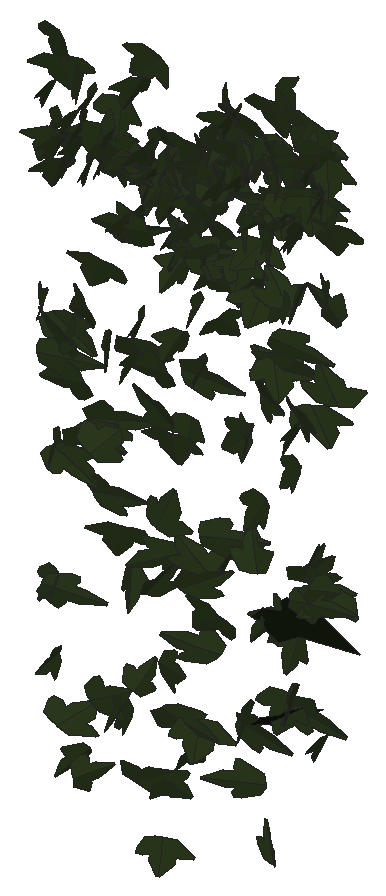
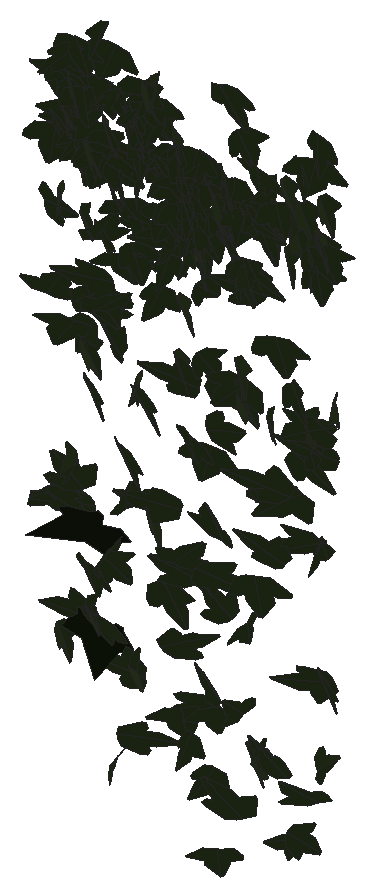
# SketchUp Ruby script. Lengths in millimetres.
U = 1.mm
M = Sketchup.active_model
def pt(a) = Geom::Point3d.new(a.map { |v| v * U })
def face(e, loops, mat)
  f = e.add_face(loops[0].map { |a| pt(a) })
  loops[1..].each { |l| e.add_face(l.map { |a| pt(a) }).erase! }
  f.material = f.back_material = mat if mat
  f
end
# faces: each face lists its corners as indices into pts; further lists are holes
def faces(e, pts, list, mat = nil) = list.each { |f| face(e, (f[0].is_a?(Array) ? f : [f]).map { |l| l.map { |i| pts[i] } }, mat) }
# xy, xz, yz: faces in a plane at the given z, y or x. An outline is a flat list of corners, or four numbers for a rectangle; further outlines are holes
def ring(l) = l.size == 4 ? [[l[0], l[1]], [l[2], l[1]], [l[2], l[3]], [l[0], l[3]]] : l.each_slice(2).to_a
def flat(e, list, mat, &to3) = list.each { |f| face(e, (f[0].is_a?(Array) ? f : [f]).map { |l| ring(l).map { |u, v| to3.(u, v) } }, mat) }
def xy(e, z, list, mat = nil) = flat(e, list, mat) { |x, y| [x, y, z] }
def xz(e, y, list, mat = nil) = flat(e, list, mat) { |x, z| [x, y, z] }
def yz(e, x, list, mat = nil) = flat(e, list, mat) { |y, z| [x, y, z] }
def lines(e, pts, list) = list.each { |a, b| e.add_line(pt(pts[a]), pt(pts[b])) }
# prism: a flat outline (further loops are holes) pulled along v
def prism(e, loops, v, mat = nil)
  f = face(e, loops, mat); d = Geom::Vector3d.new(v.map { |x| x * U })
  f.pushpull(f.normal.samedirection?(d) ? d.length : -d.length)
end
def box(e, o, s, mat = nil) = prism(e, [[o, [o[0] + s[0], o[1], o[2]], [o[0] + s[0], o[1] + s[1], o[2]], [o[0], o[1] + s[1], o[2]]]], [0, 0, s[2]], mat)
def at(x, y, z, deg = 0) = Geom::Transformation.translation(pt([x, y, z])) * Geom::Transformation.rotation(ORIGIN, Z_AXIS, deg.degrees)
def axes(o, x, y, z) = Geom::Transformation.new([*x, 0, *y, 0, *z, 0, *pt(o).to_a, 1])
def part(name) = M.definitions.add(name)
# library, detail: a bought-in or finely detailed component or shape, given as its bounding box
def library(name, o, s) = part(name).tap { |d| box(d.entities, o, s) }
def detail(e, o, s) = box(e.add_group.entities, o, s)
def put(e, d, t, mat = nil) = e.add_instance(d, t).tap { |i| i.material = mat if mat }
def group(e, t, mat = nil) = e.add_group.tap { |g| g.transformation = t; g.material = mat if mat }.entities
root = M.entities
M.materials.add("efeu1").color = [18, 25, 13]
M.materials.add("efeu2").color = [43, 57, 29]
c1 = part("ivyleaf_10")
p = [[0,12.8,-0.8],[-1.5,51.3,-10.9],[-4.9,51,-11.6],[-13.6,26.5,-7.3],[-13.2,15.9,-4.6],[-21.1,19.3,-7.2],
  [-29.5,16.3,-8.3],[-29.2,8.3,-6.2],[-19.7,-9.8,0.5],[-7.6,-13,4],[1,-12.2,5.8],[-0.4,51.1,-11.1],
  [-1.5,51.1,-10.9],[1,-12.4,5.9],[16.9,-12.4,3.5],[35.1,9.1,-5.1],[35,12.9,-6.1],[20.5,16.4,-4.9],
  [15.8,15,-3.8],[15.3,27.6,-7.1],[12.8,31.3,-7.8]]
faces(c1.entities,p,[[0,1,2,3,4,5,6,7,8,9,10],[11,12,0,13,14,15,16,17,18,19,20]],"efeu2")
c2 = part("ivyleaf_9")
p = [[39.1,54.8,31.7],[34.5,51.8,30.2],[-5.3,25.2,17.3],[-17.9,28.3,20.9],[-21.6,21.7,17],[-20.2,4.3,5.3],
  [-22.9,-0.3,2.5],[-17.1,-4,-0.6],[-2,-2.1,-1.2],[-0.7,-15.4,-10.1],[16.6,-22.3,-16.7],[21.1,-15.1,-12.5],
  [32.7,-10.7,-11],[46.1,-1.8,-6.6],[30.8,11.2,3.8]]
faces(c2.entities,p,[[0,1,2,3,4,5,6,7,8,9,10,11,12,13,14]],"efeu1")
put(root,c1,axes([1332.3,1036.5,560.2],[-0.00686,-0.08927,-0.63569],[-0.05798,0.635,-0.089],[1.22033,0.02967,-0.0078]))
put(root,c1,axes([1336.2,1057.5,753.6],[-0.73583,-0.46937,0.22543],[-0.14974,-0.22489,-0.6032],[0.97962,-0.38694,0.07713]))
put(root,c1,axes([1332.1,1056.3,814.7],[0.09283,-0.6554,-0.01014],[-0.00037,0.01015,-0.65721],[1.2475,0.04877,0.00056]))
put(root,c1,axes([1331.9,1063.9,125.8],[-0.04625,0.08812,-0.63188],[-0.26385,-0.61795,-0.08085],[-1.18521,0.13413,0.04265]))
put(root,c1,axes([1332.8,1054.4,227.3],[0.67152,-0.55596,-0.04211],[-0.04288,0.03558,-0.65847],[1.06026,0.35356,0.00004]))
put(root,c1,axes([1336.6,1057.8,771.8],[0.39508,-0.57519,-0.19],[-0.0814,0.18643,-0.61111],[1.15,0.2108,0.02202]))
put(root,c1,axes([1343.5,1052.7,726],[-0.47128,-0.6144,-0.03144],[0.02093,0.02946,-0.66242],[1.17066,-0.24787,-0.00081]))
put(root,c1,axes([1340.5,1050.9,389.7],[0.17693,-0.48285,-0.47024],[0.2146,0.47915,-0.4697],[1.26468,-0.01375,0.14549]))
put(root,c1,axes([1347.1,1047.8,757],[-0.15632,-0.66371,0.02105],[-0.00056,-0.02118,-0.66877],[1.26381,-0.08211,0.00231]))
put(root,c1,axes([1346.4,1044.7,881.1],[0.93655,-0.44172,-0.14903],[0.10035,0.26804,-0.62036],[0.88154,0.43877,0.22895]))
put(root,c1,axes([1367.5,1039.1,522.4],[-0.44439,0.33408,-0.55742],[-0.77806,0.38491,0.40194],[0.96143,0.46592,0.06763]))
put(root,c1,axes([1352.7,1048.3,851.2],[-1.13155,-0.29765,-0.08444],[0.17649,0.00307,-0.66378],[0.56176,-0.60051,0.03846]))
put(root,c1,axes([1375.6,1043.5,480.4],[-0.57648,0.07771,0.61393],[-1.16722,0.05355,-0.30936],[-0.15721,-0.68249,0.04563]))
put(root,c1,axes([1354.8,1052.8,738.9],[0.38297,-0.5402,-0.28923],[0.00625,0.30537,-0.56806],[1.16617,0.17576,0.09803]))
put(root,c1,axes([1358.2,1045.3,518.6],[0.63988,-0.5789,0.1251],[-0.11321,0.11013,0.66944],[-1.12151,-0.34141,0.00381]))
put(root,c1,axes([1365.8,1049.1,792.1],[-0.02554,-0.65638,0.0168],[-0.01007,-0.01669,-0.6565],[1.2496,-0.01355,-0.00495]))
put(root,c1,axes([1366.6,1061.7,25.4],[-0.0766,-0.43309,0.47651],[-0.0449,-0.47613,-0.43473],[1.22468,-0.04454,0.01386]))
put(root,c1,axes([1341.7,1048.7,220.6],[-0.28811,-0.09888,-0.63937],[1.1804,0.16469,-0.17232],[0.35041,-0.63607,0.05477]))
put(root,c1,axes([1343.2,1056.3,534.8],[0.90612,0.09577,0.47932],[0.86018,0.16854,-0.48261],[-0.35425,0.65422,0.05416]))
put(root,c1,axes([1339.2,1046.5,498.4],[0.19337,-0.05206,-0.67101],[1.27587,-0.0523,0.10556],[-0.11349,-0.67664,0.04347]))
put(root,c1,axes([1381,1050.2,566.6],[-0.56102,0.23975,0.51389],[-0.84038,0.26634,-0.37754],[-0.67714,-0.52919,0.0428]))
put(root,c1,axes([1372.9,1050.3,761.5],[-0.05381,-0.65385,-0.01163],[-0.01269,0.01193,-0.65443],[1.24455,-0.02815,-0.00717]))
put(root,c1,axes([1357.6,1045.7,68.6],[0.87358,0.11605,-0.44595],[0.67555,0.31233,0.44663],[0.55924,-0.55857,0.15709]))
put(root,c1,axes([1354.6,1044.4,385.3],[0.79663,0.19512,0.47103],[0.81579,0.19531,-0.46181],[-0.52541,0.59911,-0.00286]))
put(root,c1,axes([1377.4,1043.1,841.4],[0.54888,-0.57359,-0.24048],[-0.04153,0.25558,-0.63578],[1.18299,0.27511,0.08925]))
put(root,c1,axes([1380.4,1041.2,787],[-0.03679,-0.49141,-0.47177],[0.08739,0.46995,-0.49139],[1.29354,-0.04572,0.01978]))
put(root,c1,axes([1380.1,1057.1,736.3],[0.28652,-0.62247,-0.10999],[0.05396,0.1196,-0.63806],[1.20182,0.14303,0.05487]))
put(root,c1,axes([1383.4,1056.8,819],[0.25412,-0.64214,-0.01462],[-0.01335,0.01347,-0.65586],[1.22237,0.13364,-0.00412]))
put(root,c1,axes([1397.3,1056.8,620.3],[-1.15263,-0.08738,0.19608],[-0.36259,-0.05166,-0.61147],[0.18826,-0.63448,0.02279]))
put(root,c1,axes([1379,1044.6,11.4],[0.07847,0.04993,-0.655],[0.61551,0.5697,0.06379],[1.0882,-0.32583,0.01115]))
put(root,c1,axes([1398.4,1053.5,783.8],[-0.78386,-0.51185,0.09508],[0.05626,-0.14403,-0.64733],[0.98922,-0.3974,0.11216]))
put(root,c1,axes([1388.5,1040.3,427],[-0.79844,-0.26297,-0.51972],[0.84591,0.26942,-0.4951],[0.71645,-0.61117,0.00537]))
put(root,c1,axes([1406.6,1044.4,758],[0.3273,-0.5681,-0.25628],[0.01322,0.26759,-0.58851],[1.18607,0.15379,0.07728]))
put(root,c1,axes([1398.6,1065.4,528.8],[0.425,-0.52002,0.29566],[0.40747,-0.2252,-0.5578],[1.06306,0.29422,0.0956]))
put(root,c1,axes([1416.6,1053.4,753.1],[0.87223,-0.29069,-0.36046],[-0.32277,0.36655,-0.51122],[0.82009,0.45344,0.18218]))
put(root,c1,axes([1392.2,1060.8,99.8],[0.82859,-0.19174,-0.44873],[0.762,-0.20342,0.47538],[-0.53093,-0.59121,-0.01803]))
put(root,c1,axes([1407.6,1035,417.3],[0.55694,0.2796,-0.64011],[0.62537,0.55732,0.39366],[1.17312,-0.42984,0.09404]))
put(root,c1,axes([1442.8,1055.9,764.5],[-0.12836,0.12528,0.62325],[-1.2046,0.04537,-0.07761],[-0.11313,-0.62524,0.11925]))
put(root,c1,axes([1427.5,1055.3,313.8],[-1.04517,-0.37019,0.07828],[-0.12379,-0.04356,-0.66228],[0.7094,-0.553,-0.00024]))
put(root,c1,axes([1401.5,1053.4,438.2],[-0.36839,-0.16323,0.66632],[0.98798,0.41776,0.25314],[-0.85356,0.554,0.00543]))
put(root,c1,axes([1421.4,1034.9,796.7],[-0.02991,-0.03598,-0.69138],[0.26434,0.67733,-0.03841],[1.29082,-0.13954,-0.00815]))
put(root,c1,axes([1420.3,1058.6,100],[0.15907,-0.19679,0.62358],[0.39507,-0.58815,-0.21343],[1.18012,0.22342,-0.0126]))
put(root,c1,axes([1404.6,1049.6,353.1],[-0.50568,-0.03052,0.58921],[1.10998,0.08414,0.26735],[-0.16981,0.64085,-0.00704]))
put(root,c1,axes([1422,1044.4,777.7],[-0.68013,-0.43856,-0.36402],[0.43322,0.28409,-0.56572],[0.99447,-0.42369,-0.00252]))
put(root,c1,axes([1435.2,1052.3,102.8],[0.50005,-0.5423,-0.26097],[-0.20438,0.23794,-0.60257],[1.12702,0.28377,0.00652]))
put(root,c1,axes([1455.3,1045.9,687.6],[-0.41925,-0.00398,0.66367],[-1.25886,-0.05607,-0.21989],[0.10366,-0.69702,0.0139]))
put(root,c1,axes([1423.7,1052.5,821.2],[1.16308,-0.26994,0.16014],[0.26839,-0.07699,-0.66795],[0.53365,0.62704,-0.01308]))
put(root,c1,axes([1438.9,1052.8,691],[-0.23653,-0.64738,-0.0655],[0.01686,0.065,-0.65919],[1.23826,-0.12454,-0.00354]))
put(root,c1,axes([1415,1049.3,757.9],[-0.44416,0.07954,-0.60477],[1.06648,-0.22786,-0.2462],[-0.45865,-0.60687,0.01317]))
put(root,c1,axes([1437,1059.4,261.7],[0.12007,0.64123,-0.31004],[-0.1205,-0.30497,-0.64364],[-1.35019,0.08424,0.02987]))
put(root,c1,axes([1443.5,1055.1,698],[-0.32129,-0.60605,-0.25],[0.13768,0.23936,-0.6291],[1.24009,-0.18359,0.00507]))
put(root,c1,axes([1447.6,1053.3,856.4],[-0.33131,-0.62171,0.15575],[-0.02896,-0.15734,-0.64506],[1.21946,-0.17265,0.027]))
put(root,c1,axes([1443.3,1054.2,760.9],[-0.74897,-0.50942,-0.15101],[0.27774,0.07706,-0.64027],[0.97234,-0.4144,0.06657]))
put(root,c1,axes([1446.6,1052.1,531],[0.15266,-0.60947,0.22363],[0.04973,-0.22211,-0.61472],[1.23457,0.08431,-0.00289]))
put(root,c1,axes([1449.3,1055.5,574.8],[0.20397,-0.62045,-0.16683],[-0.01936,0.16748,-0.62939],[1.22263,0.10616,0.01786]))
put(root,c1,axes([1431.4,1052.7,672],[-0.11162,-0.34172,0.53698],[0.67526,0.43015,0.31248],[-1.0057,0.32674,0.15022]))
put(root,c1,axes([1452.9,1047.3,143.9],[0.30692,0.38769,-0.48276],[0.37266,0.44133,0.41983],[1.11791,-0.25356,-0.00741]))
put(root,c1,axes([1461.6,1055.5,742.7],[0.36603,-0.6045,-0.13853],[0.06646,0.15536,-0.62948],[1.17844,0.179,0.07853]))
put(root,c1,axes([1452.5,1048.8,546.1],[-1.19271,0.08538,-0.31229],[0.58647,-0.05139,-0.63242],[-0.18898,-0.6983,0.00836]))
put(root,c1,axes([1463.7,1045.1,786.7],[-0.29152,-0.57233,-0.33623],[0.17215,0.32385,-0.59247],[1.25154,-0.17786,0.00318]))
put(root,c1,axes([1469.3,1059.9,750.2],[-0.58038,-0.55748,0.12489],[0.01226,-0.14492,-0.63113],[1.08722,-0.29596,0.07379]))
put(root,c1,axes([1462.9,1063.4,734.3],[0.74107,-0.48932,0.14193],[0.16888,-0.11077,-0.62534],[0.95484,0.39936,0.00045]))
put(root,c1,axes([1488.6,1041.8,533],[-0.50398,0.0617,0.60507],[-1.13825,0.09356,-0.27128],[-0.21044,-0.65382,0.01827]))
put(root,c1,axes([1469.7,1054.8,793.7],[0.41106,-0.59554,-0.18444],[-0.0672,0.1832,-0.63287],[1.18463,0.21704,0.0281]))
put(root,c1,axes([1474.9,1044.3,897.7],[1.05169,-0.26567,-0.34608],[-0.45899,0.2794,-0.59957],[0.69197,0.58912,0.12829]))
put(root,c1,axes([1472.4,1057.6,752.4],[-0.3491,-0.62597,0.04653],[-0.03518,-0.04307,-0.65227],[1.19411,-0.18427,-0.00561]))
put(root,c1,axes([1455.2,1056,26],[-0.92702,-0.19327,0.39528],[0.70381,0.13972,0.524],[-0.45377,0.61154,0.00521]))
put(root,c1,axes([1491.8,1042.2,476.2],[-0.53705,0.20796,-0.5476],[-0.81467,0.34171,0.35035],[0.76099,0.51257,-0.01139]))
put(root,c1,axes([1476.1,1057.9,767.1],[0.10141,-0.6501,-0.05822],[-0.01499,0.05777,-0.65228],[1.24214,0.05377,-0.00312]))
put(root,c1,axes([1480.4,1055.4,749.7],[-0.79794,-0.40959,0.25796],[-0.15047,-0.27875,-0.57109],[0.90888,-0.40574,0.13193]))
put(root,c1,axes([1489.1,1059.7,306.5],[-0.42664,-0.25606,0.61545],[-0.58968,-0.53489,-0.3354],[1.12328,-0.37805,0.05768]))
put(root,c1,axes([1472.2,1051.6,262.5],[-0.14374,-0.60993,0.28193],[0.0693,0.27957,0.61458],[-1.27695,0.08383,0.00162]))
put(root,c1,axes([1487.9,1063.3,728.6],[-0.30697,-0.60038,0.14721],[-0.03151,-0.14788,-0.62129],[1.17607,-0.16067,0.02178]))
put(root,c1,axes([1482.5,1051,-39.4],[0.8563,0.44593,-0.07956],[-0.11736,-0.0508,-0.63343],[-0.85408,0.45408,0.00727]))
put(root,c1,axes([1492.7,1052.8,783.8],[0.45627,-0.59477,0.09252],[0.04733,-0.08971,-0.64118],[1.14459,0.2408,-0.01037]))
put(root,c1,axes([1477.4,1065.7,166.1],[0.16267,-0.18588,-0.63532],[0.62281,-0.54498,0.20348],[-1.09513,-0.33754,0.02135]))
put(root,c1,axes([1495.9,1051.3,450.6],[-1.21277,-0.02421,-0.01622],[0.03089,-0.00002,-0.63769],[0.04606,-0.63743,0.00063]))
put(root,c1,axes([1496.1,1054.8,740.2],[0.35355,-0.58758,-0.16925],[0.01696,0.17947,-0.61328],[1.16362,0.17591,0.06036]))
put(root,c1,axes([1486.8,1046.2,351.5],[1.20432,-0.35767,-0.06101],[0.11766,-0.01458,0.72666],[-0.68045,-0.63555,0.01767]))
put(root,c1,axes([1497.5,1057.8,568.8],[-0.27937,-0.50179,0.37147],[0.09764,-0.39,-0.50655],[1.18419,-0.08622,0.1294]))
put(root,c1,axes([1498.9,1057.2,655.8],[-0.31972,-0.36698,0.51188],[0.22237,-0.53874,-0.34789],[1.1779,0.0021,0.20462]))
put(root,c1,axes([1502.4,1047,702.2],[0.06894,-0.59354,-0.25176],[0.05631,0.25342,-0.5932],[1.22575,0.02174,0.04141]))
put(root,c1,axes([1495.5,1051.9,806.6],[-0.98716,0.3402,-0.19325],[0.29031,-0.11968,-0.6201],[-0.68572,-0.54042,0.01567]))
put(root,c1,axes([1502,1041.8,793.2],[0.36663,0.60685,0.10715],[-0.20021,0.143,-0.62076],[-1.15562,0.16775,0.14154]))
put(root,c1,axes([1499.7,1040.5,47],[-0.43307,-0.44365,-0.43111],[0.45879,0.35945,-0.49714],[1.08427,-0.32929,0.03816]))
put(root,c1,axes([1500.4,1046.2,792.3],[-0.03249,0.63833,-0.12351],[0.02033,-0.12326,-0.63852],[-1.23723,-0.01879,-0.00725]))
put(root,c1,axes([1509.9,1050.3,686.3],[0.39484,-0.57715,-0.18427],[-0.06742,0.18289,-0.61269],[1.15108,0.20868,0.02732]))
put(root,c1,axes([1510.6,1036.9,672.9],[0.51034,-0.36345,0.57601],[-0.45291,0.53003,0.44522],[-1.21455,-0.35037,0.076]))
put(root,c1,axes([1506.3,1054,776.9],[1.22294,0.11943,0.00816],[-0.00731,0.0651,-0.65037],[-0.22771,0.63932,0.0647]))
put(root,c1,axes([1509.8,1059.3,761.6],[0.81436,-0.48623,0.05749],[0.15634,-0.00397,-0.64502],[0.91863,0.43172,0.05881]))
put(root,c1,axes([1517.3,1050.3,807.3],[-1.18894,0.18782,0.04065],[-0.07439,0.0112,-0.65233],[-0.35809,-0.62593,0.00053]))
put(root,c1,axes([1507.1,1063.3,465.6],[1.02582,-0.35639,0.20084],[0.31834,-0.11118,-0.64617],[0.71051,0.56436,-0.00046]))
put(root,c1,axes([1522.2,1050.4,741],[-1.02527,0.31995,0.11542],[-0.24543,0.00792,-0.62386],[-0.59901,-0.55088,0.05806]))
put(root,c1,axes([1532.3,1064.2,205.3],[0.27797,0.31587,0.61204],[-0.55052,-0.53967,0.34754],[1.18961,-0.32355,0.01782]))
put(root,c1,axes([1503.6,1042.7,128.8],[-0.82742,-0.05458,-0.5217],[0.97999,0.08485,-0.43797],[0.19044,-0.67378,-0.0129]))
put(root,c1,axes([1520.6,1051.7,86.5],[-0.1856,-0.47273,-0.46587],[0.22044,0.45153,-0.48242],[1.24379,-0.15057,0.01598]))
put(root,c1,axes([1522.5,1058,758.1],[0.52452,-0.58774,-0.07754],[0.02356,0.0912,-0.64726],[1.12804,0.27138,0.04957]))
put(root,c1,axes([1537.9,1041.9,690.6],[0.95335,0.00863,0.51223],[-0.96947,0.08467,0.49672],[-0.10382,-0.71143,0.06533]))
put(root,c1,axes([1521.3,1057.7,777.2],[1.0362,0.33969,-0.08162],[-0.15284,-0.02539,-0.64139],[-0.64709,0.54995,0.0208]))
put(root,c1,axes([1529.9,1057.6,308.8],[0.80325,0.40958,0.25548],[-0.34746,-0.17872,0.58812],[0.85049,-0.45985,-0.00102]))
put(root,c1,axes([1524.2,1049.2,688],[0.09501,-0.38401,-0.51185],[0.1175,0.5139,-0.37953],[1.21214,-0.01972,0.07691]))
put(root,c1,axes([1524.3,1042.8,716],[-0.39327,-0.53988,-0.30294],[0.25629,0.27252,-0.57753],[1.14999,-0.24536,0.02511]))
put(root,c1,axes([1529.4,1058.6,740.2],[-0.74614,-0.51318,0.08154],[0.06449,-0.12718,-0.63748],[0.98682,-0.3797,0.10331]))
put(root,c1,axes([1528.5,1053.8,621.7],[0.42056,-0.60664,-0.00253],[-0.00166,0.00238,-0.64563],[1.15457,0.22098,-0.00001]))
put(root,c1,axes([1532.1,1053.3,793.2],[-0.27681,-0.63951,0.10688],[0.00076,-0.10962,-0.65539],[1.23399,-0.14339,0.02438]))
put(root,c1,axes([1538.9,1052.5,803.4],[-0.76857,0.39671,0.35406],[-0.5682,0.19874,-0.5632],[-0.83742,-0.49894,0.05718]))
put(root,c1,axes([1535.1,1054.3,762.3],[-1.08496,-0.29009,0.06256],[-0.09396,-0.0409,-0.63948],[0.55692,-0.57204,0.01399]))
put(root,c1,axes([1536.9,1046.4,783.6],[-1.21714,-0.08182,0.08241],[-0.13865,-0.07655,-0.64133],[0.17211,-0.64025,0.06615]))
put(root,c1,axes([1535.1,1051.9,550.5],[0.29222,-0.61507,-0.08584],[-0.02875,0.0847,-0.63392],[1.1816,0.15417,0.00581]))
put(root,c1,axes([1531.1,1051.8,117.1],[0.95925,0.52673,-0.12343],[-0.16525,-0.08775,-0.72903],[-1.01628,0.51144,0.00204]))
put(root,c1,axes([1526,1047,286.5],[-0.40369,-0.39566,0.52059],[0.46139,0.46071,0.44892],[-1.15578,0.32211,-0.00262]))
put(root,c1,axes([1539.3,1052.6,820.2],[0.41757,-0.62079,-0.10657],[0.00846,0.11437,-0.6571],[1.19875,0.21544,0.04176]))
put(root,c1,axes([1554.5,1049.9,258],[-1.0311,0.07274,0.41151],[-0.77757,0.04941,-0.54662],[-0.16716,-0.67854,0.00431]))
put(root,c1,axes([1541.4,1059.8,740.1],[-0.48053,-0.59193,0.08358],[0.03431,-0.09823,-0.64121],[1.13723,-0.24715,0.05466]))
put(root,c1,axes([1519,1058.2,531.6],[-0.11178,-0.04999,0.68185],[1.27448,0.13374,0.06749],[-0.26228,0.67118,0.03734]))
put(root,c1,axes([1551,1049.1,797.5],[-0.7285,-0.5273,0.0378],[-0.04062,-0.03121,-0.65159],[1.00531,-0.38337,0.00106]))
put(root,c1,axes([1552.4,1041.2,681.4],[-0.04706,0.03408,0.67814],[-0.42835,0.63981,-0.04036],[-1.2192,-0.2261,-0.01199]))
put(root,c1,axes([1554.1,1052.9,782.8],[-0.63263,-0.57437,0.05078],[0.05003,-0.07365,-0.66095],[1.09627,-0.32809,0.05947]))
put(root,c1,axes([1549.8,1051.7,666.9],[-0.28518,-0.53214,-0.32558],[0.27987,0.29527,-0.55029],[1.15383,-0.20314,0.05301]))
put(root,c1,axes([1547.5,1044.1,772.9],[0.1432,0.3696,0.54415],[0.02826,0.54661,-0.37332],[-1.25161,0.05463,0.05383]))
put(root,c1,axes([1554.7,1052.9,723.3],[-1.07765,0.29359,-0.00032],[0.00092,0.00023,-0.63782],[-0.55877,-0.56623,-0.00042]))
put(root,c1,axes([1557.1,1052,834.1],[0.17151,0.55236,-0.35938],[-0.23677,-0.34194,-0.55675],[-1.23161,0.14266,0.05699]))
put(root,c1,axes([1553.4,1047.9,798.8],[-0.41123,-0.49266,-0.36988],[0.47209,0.28922,-0.53013],[1.07323,-0.31599,0.09146]))
put(root,c1,axes([1563,1043,780.7],[-0.12262,-0.59383,-0.28635],[0.14057,0.2794,-0.59604],[1.24682,-0.0899,0.03904]))
put(root,c1,axes([1546.1,1036.1,686.6],[0.083,-0.11778,0.71708],[0.71594,0.61829,0.07868],[-1.18331,0.36583,0.0979]))
put(root,c1,axes([1561,1054.3,787.8],[1.26105,-0.01612,-0.00916],[-0.01732,0.00268,-0.66279],[0.03075,0.66265,0.00246]))
put(root,c1,axes([1574.9,1044.7,879.1],[-0.51893,0.39824,0.45446],[-0.49484,0.37274,-0.48263],[-1.03812,-0.37675,0.00288]))
put(root,c1,axes([1574.5,1051.4,852.9],[1.17661,0.04994,-0.24838],[-0.4783,0.20381,-0.58455],[0.06105,0.63432,0.20737]))
put(root,c1,axes([1566.9,1044.5,619.6],[-0.48117,-0.46382,-0.38639],[0.33399,0.34435,-0.52818],[1.0993,-0.30763,-0.00865]))
put(root,c1,axes([1576.1,1049,343.9],[0.23806,-0.64797,-0.11141],[-0.05172,0.10822,-0.65991],[1.25025,0.12786,-0.00608]))
put(root,c1,axes([1566.8,1058.3,795],[0.96799,-0.37359,0.17246],[0.26684,-0.10045,-0.63107],[0.73627,0.52758,0.00197]))
put(root,c1,axes([1594.2,1061.4,70.1],[-0.08567,0.05779,0.66251],[-0.73657,-0.54227,0.021],[1.02926,-0.38325,0.07017]))
put(root,c1,axes([1579.8,1050.1,866.8],[0.15119,-0.65598,0.04507],[0.01761,-0.04428,-0.66076],[1.25127,0.07988,0.00385]))
put(root,c1,axes([1590.3,1050.4,487.5],[0.70798,-0.51984,-0.35564],[-0.40707,0.28423,-0.63918],[1.12749,0.42904,-0.00746]))
put(root,c1,axes([1581.2,1050.3,830],[-0.99993,-0.35416,-0.188],[0.26885,0.12652,-0.63313],[0.7142,-0.54349,-0.02488]))
put(root,c1,axes([1558,1043.5,359],[0.16066,0.01855,-0.6977],[1.28139,0.183,0.08633],[0.34999,-0.67854,0.00421]))
put(root,c1,axes([1588.3,1049.6,866.3],[-1.15815,0.26913,0.0819],[-0.12835,0.04992,-0.66513],[-0.51979,-0.61198,-0.01824]))
put(root,c1,axes([1592.7,1056.8,666.7],[-0.48396,-0.62194,0.03039],[-0.02126,-0.02826,-0.67192],[1.1849,-0.25453,0.00035]))
put(root,c1,axes([1592.1,1051.3,796.1],[-0.2062,-0.62211,-0.16859],[0.02771,0.16855,-0.63131],[1.22639,-0.10841,-0.01408]))
put(root,c1,axes([1585.6,1048.1,695.7],[1.23197,-0.0105,0.03973],[0.0757,0.00237,-0.64739],[0.01967,0.64853,0.003]))
put(root,c1,axes([1596.1,1052.8,820.4],[0.50026,-0.58889,-0.16814],[-0.07999,0.1652,-0.64428],[1.16282,0.26471,0.02802]))
put(root,c1,axes([1589,1061.2,154.7],[0.33861,-0.40227,0.52736],[0.42874,-0.4769,-0.43978],[1.18731,0.28693,0.00841]))
put(root,c1,axes([1593.6,1048.6,837.1],[0.01195,0.67482,-0.04731],[-0.01149,-0.04725,-0.67483],[-1.28742,0.00669,0.00558]))
put(root,c1,axes([1601.4,1040.1,494.3],[0.17182,-0.14104,-0.66146],[-0.02007,0.66695,-0.14365],[1.28703,0.02923,0.08606]))
put(root,c1,axes([1590,1055.4,744.6],[0.17355,-0.47855,0.4245],[0.55864,-0.34968,-0.45726],[1.08173,0.25737,0.16804]))
put(root,c1,axes([1608.8,1052.7,717.5],[0.95264,0.26687,-0.30251],[-0.51917,-0.13124,-0.56713],[-0.5656,0.56995,0.01106]))
put(root,c1,axes([1606,1059.1,655],[1.05274,0.38276,-0.16418],[-0.24602,-0.1017,-0.67259],[-0.75352,0.56796,-0.00978]))
put(root,c1,axes([1609.3,1045.4,344.5],[0.2897,0.70501,-0.21929],[0.08569,0.21462,0.72125],[1.40256,-0.15873,0.00123]))
put(root,c1,axes([1611.3,1051.7,411.9],[0.88865,-0.55762,-0.06008],[-0.06749,0.04866,-0.72728],[1.06526,0.46825,0.00404]))
put(root,c1,axes([1618.6,1058.4,761.4],[-0.1592,-0.45227,0.45421],[-0.2021,-0.44196,-0.45962],[1.20306,-0.13409,-0.0171]))
put(root,c1,axes([1607.1,1049.8,832.2],[0.91795,-0.46295,0.05336],[0.23049,0.05037,-0.65772],[0.85645,0.48264,0.11982]))
put(root,c1,axes([1614.6,1048.1,832.7],[0.54194,-0.59519,-0.0542],[-0.03445,0.05142,-0.65978],[1.13694,0.28527,0.00584]))
put(root,c1,axes([1619.5,1064.5,276.7],[-0.21242,-0.50792,0.38042],[-0.0352,-0.38349,-0.51745],[1.20724,-0.10055,0.05185]))
put(root,c1,axes([1626.3,1046.7,744.5],[0.21824,-0.29115,-0.5829],[-0.36632,0.55031,-0.31273],[1.18473,0.22379,0.01068]))
put(root,c1,axes([1642.9,1052.2,781],[0.15637,0.10062,-0.64304],[-1.22595,-0.08031,-0.09487],[-0.1775,0.64328,0.08874]))
put(root,c1,axes([1597.5,1049.6,141.9],[0.07581,-0.10485,0.68744],[1.3228,-0.01578,-0.04268],[0.04186,0.68841,0.10373]))
put(root,c1,axes([1624.5,1048.7,847.3],[0.31361,0.65327,-0.02323],[-0.12879,-0.00678,-0.67069],[-1.2374,0.16627,0.06392]))
put(root,c1,axes([1621.2,1058.7,735.7],[0.56151,-0.48495,0.30679],[0.39774,-0.23047,-0.56529],[1.01713,0.35784,0.05169]))
put(root,c1,axes([1636.8,1037.4,9.4],[-0.09233,0.4928,-0.44903],[-0.13681,0.44373,0.49474],[1.26145,0.08419,0.02079]))
put(root,c1,axes([1629.4,1066.6,271.3],[-0.25494,0.38373,0.64136],[0.3082,-0.6212,0.40549],[1.38864,0.20832,0.02775]))
put(root,c1,axes([1632.5,1047.6,896],[-1.2709,0.09926,-0.07014],[0.12785,-0.025,-0.67495],[-0.19278,-0.67098,0.01477]))
put(root,c1,axes([1632.1,1053.2,804],[0.65192,-0.57038,-0.01055],[0.06128,0.03162,-0.66388],[1.084,0.34124,0.04388]))
put(root,c1,axes([1614.4,1055.1,539.1],[-0.32926,0.10333,0.67463],[1.08026,-0.36467,0.20141],[0.72127,0.59335,0.00631]))
put(root,c1,axes([1641.4,1055.2,577.6],[0.63807,0.43245,0.34069],[-0.39164,-0.27154,0.54718],[0.97181,-0.39337,-0.00318]))
put(root,c1,axes([1652.8,1053.6,591.9],[-0.95019,-0.31226,0.34526],[-0.54298,-0.19481,-0.58875],[0.7001,-0.5749,0.01198]))
put(root,c1,axes([1627.8,1052.8,774.7],[1.14806,0.21911,0.16144],[0.29261,0.04958,-0.64176],[-0.42742,0.62249,-0.00572]))
put(root,c1,axes([1638.1,1057.4,763.9],[-0.88722,-0.43377,-0.11788],[0.27679,0.01515,-0.63087],[0.80948,-0.48061,0.08651]))
put(root,c1,axes([1643.1,1051.9,668.4],[0.55904,0.60761,0.09095],[-0.08636,-0.07908,0.67485],[1.16609,-0.29715,0.00637]))
put(root,c1,axes([1636.8,1052,843.4],[0.0447,0.60291,-0.28232],[-0.01767,-0.28217,-0.60336],[-1.2669,0.02521,-0.00154]))
put(root,c1,axes([1645.7,1047.9,668.7],[0.68767,-0.5316,-0.13386],[-0.12626,0.11675,-0.64268],[1.03566,0.36721,0.01054]))
put(root,c1,axes([1637.1,1046.3,587],[0.85427,0.5418,-0.00013],[-0.01047,0.00439,-0.70355],[-1.03111,0.44884,0.00704]))
put(root,c2,axes([1647.7,1042.1,177.2],[0.50458,0.7127,0.07502],[0.04728,0.0708,-0.76042],[-1.36309,0.26628,0.00139]))
put(root,c1,axes([1636.5,1047.3,845.9],[-1.05005,0.22528,-0.30258],[0.51666,-0.13514,-0.59561],[-0.49851,-0.61457,0.02005]))
put(root,c1,axes([1646.5,1046.7,919],[-0.08066,0.56585,0.36736],[-0.24589,0.35447,-0.56089],[-1.26021,-0.10538,0.08593]))
put(root,c1,axes([1652.5,1058.3,776.3],[0.15828,-0.64572,0.0393],[-0.00547,-0.03999,-0.65101],[1.2312,0.08283,-0.00794]))
put(root,c1,axes([1651.6,1054.6,765.2],[-0.594,-0.53525,-0.20674],[0.18955,0.18123,-0.61958],[1.07546,-0.32757,-0.00498]))
put(root,c1,axes([1647.3,1050.8,189.9],[1.27085,-0.28628,0.03483],[0.06093,-0.01373,-0.72652],[0.54547,0.66851,0]))
put(root,c1,axes([1651.3,1060.4,257.9],[1.03738,-0.43776,0.08882],[0.14007,-0.0502,-0.69906],[0.8385,0.54998,0.00689]))
put(root,c1,axes([1661.4,1047.2,473.7],[0.63099,-0.55712,-0.18708],[-0.17282,0.16365,-0.64829],[1.10506,0.34371,0.00543]))
put(root,c1,axes([1654.6,1054.5,201.8],[0.45686,-0.57595,0.31996],[0.29795,-0.28092,-0.62313],[1.21803,0.28475,0.03242]))
put(root,c1,axes([1662.4,1046.1,758.2],[0.24943,-0.62894,-0.11532],[-0.06677,0.11047,-0.64235],[1.21512,0.13517,-0.01162]))
put(root,c1,axes([1662,1052.1,521.9],[0.1975,-0.6811,0.11836],[0.01202,-0.11875,-0.68887],[1.31565,0.10333,-0.01148]))
put(root,c1,axes([1666.8,1051.2,831.8],[-0.96589,-0.42588,0.04296],[-0.04494,-0.03868,-0.66237],[0.81341,-0.50785,0.01442]))
put(root,c1,axes([1667.5,1052.9,760.3],[0.10689,-0.64726,0.09818],[-0.01311,-0.09912,-0.64952],[1.24589,0.05449,-0.01526]))
put(root,c1,axes([1646.2,1047.9,789.3],[0.58479,0.26062,0.59411],[0.71626,0.46386,-0.39812],[-1.00574,0.48189,0.06192]))
put(root,c1,axes([1674.6,1049.2,839.4],[-0.91563,-0.41426,0.20769],[-0.2506,-0.16484,-0.6338],[0.84562,-0.49741,0.03707]))
put(root,c1,axes([1642.2,1055.2,614.8],[-0.30341,0.0089,-0.64339],[1.21404,-0.08478,-0.15923],[-0.16067,-0.65741,0.01183]))
put(root,c1,axes([1666.6,1045.8,545],[-0.90275,0.45423,0.01807],[-0.02642,0.01164,-0.65674],[-0.86476,-0.47453,0.0012]))
put(root,c1,axes([1663.9,1052.9,682.4],[0.43497,-0.52585,0.28258],[0.24747,-0.25147,-0.57312],[1.10888,0.26239,0.01706]))
put(root,c1,axes([1679.9,1049.1,888.5],[-1.17898,0.2017,0.17565],[-0.42802,-0.15298,-0.61749],[-0.27551,-0.62545,0.20768]))
put(root,c1,axes([1669.9,1044.5,774.5],[-0.22371,-0.29919,-0.63473],[0.43338,0.59248,-0.32145],[1.26322,-0.25625,-0.00213]))
put(root,c2,axes([1653.4,1042.5,301.7],[0.09154,-0.09955,-0.7675],[0.681,0.68471,-0.06639],[1.30605,-0.35005,0.08841]))
put(root,c1,axes([1684.5,1048.6,842.7],[0.13132,-0.6441,-0.16655],[-0.0254,0.16607,-0.64777],[1.26591,0.07015,0.00428]))
put(root,c1,axes([1687.7,1045.4,367.3],[0.12762,-0.14594,0.67639],[-0.5078,0.62155,0.16056],[-1.21509,-0.27508,0.00394]))
put(root,c1,axes([1679.4,1049.1,350.8],[-0.60862,-0.5378,0.23744],[0.26077,0.19467,0.62546],[-1.08805,0.34749,0.01709]))
put(root,c1,axes([1682,1048.3,794.8],[1.151,0.26069,0.04446],[-0.00568,0.1177,-0.64948],[-0.50327,0.59487,0.10902]))
put(root,c1,axes([1683.8,1050,804.9],[1.18295,0.19311,0.12015],[0.0689,0.26119,-0.60707],[-0.42734,0.57667,0.23473]))
put(root,c1,axes([1693.5,1048.6,854.1],[-0.65707,-0.56999,-0.08475],[0.09709,0.06818,-0.66635],[1.09243,-0.3489,0.00825]))
put(root,c1,axes([1693.3,1051.3,808.3],[0.40648,-0.61791,0.11175],[0.0274,-0.11319,-0.65338],[1.19478,0.21282,-0.02304]))
put(root,c1,axes([1696,1052.9,161.8],[0.07039,-0.64776,-0.02521],[0.0007,0.02527,-0.64881],[1.23374,0.03694,0.00181]))
put(root,c1,axes([1666.8,1047,188.4],[0.21778,-0.04758,0.69596],[1.32091,0.07871,-0.10873],[-0.13355,0.7009,0.05946]))
put(root,c1,axes([1703.1,1060.3,331.4],[0.90934,0.29842,-0.4379],[-0.70291,-0.23529,-0.56332],[-0.72324,0.60389,-0.00309]))
put(root,c1,axes([1683.3,1053.5,544.6],[1.03975,0.30182,0.21961],[0.35267,0.11861,-0.624],[-0.61666,0.57673,0.01341]))
put(root,c1,axes([1698.6,1043,816.5],[0.61268,-0.50495,-0.29194],[-0.01797,0.3289,-0.57929],[1.10994,0.28406,0.15177]))
put(root,c1,axes([1704.1,1045.3,694.1],[0.07617,-0.10856,-0.66867],[-0.14065,0.66514,-0.11241],[1.28158,0.07945,0.0274]))
put(root,c1,axes([1675.7,1044.7,321.7],[-0.07351,-0.03541,-0.64209],[1.21212,0.08686,-0.0431],[0.16926,-0.63736,0.0298]))
put(root,c1,axes([1690.3,1046.3,874.3],[-0.39223,-0.40817,-0.49563],[0.65216,0.37028,-0.44743],[1.03341,-0.3886,0.09425]))
put(root,c1,axes([1718.8,1045.8,678.4],[0.44001,-0.09019,0.62127],[-1.11382,0.20861,0.24807],[-0.43235,-0.62921,-0.0068]))
put(root,c1,axes([1691.8,1049,339.8],[-0.22011,-0.19552,-0.63132],[0.73225,0.5012,-0.2257],[1.02272,-0.40093,0.02573]))
put(root,c1,axes([1703.8,1053.1,792.8],[0.7514,-0.52936,-0.00765],[-0.02166,0.00105,-0.66032],[1.00735,0.39488,-0.00849]))
put(root,c1,axes([1706.9,1053.6,772.8],[-1.21097,-0.16446,-0.02013],[0.03136,0.0167,-0.65708],[0.31378,-0.63638,-0.01204]))
put(root,c1,axes([1700.8,1050.4,847.2],[1.2335,-0.04807,0.13555],[0.2578,-0.00625,-0.64989],[0.09199,0.66211,0.0037]))
put(root,c1,axes([1712.6,1050.6,575.8],[1.0891,0.27682,0.15029],[-0.26343,-0.05897,0.63565],[0.5385,-0.58871,0.007]))
